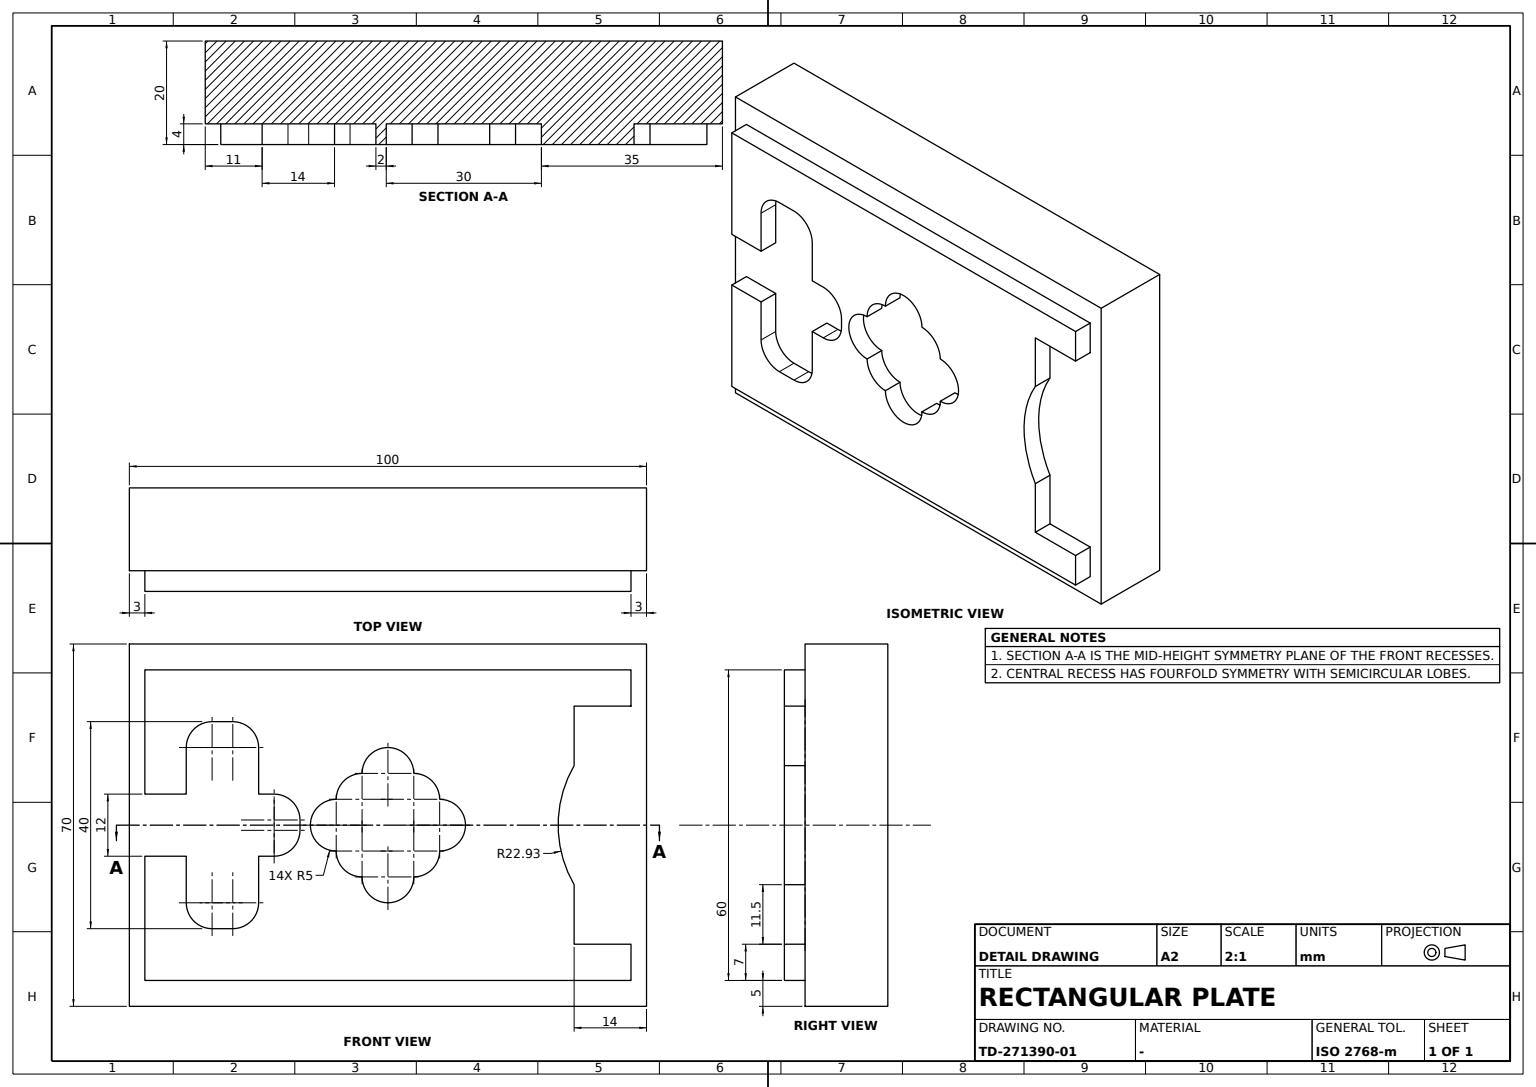
ISO-10303-21;
HEADER;
FILE_DESCRIPTION((''),'2;1');
FILE_NAME('','',(''),(''),'','','');
FILE_SCHEMA(('AUTOMOTIVE_DESIGN'));
ENDSEC;
DATA;
#1=APPLICATION_CONTEXT('');
#2=PRODUCT_CONTEXT('',#1,'mechanical');
#3=PRODUCT('','','',(#2));
#4=PRODUCT_DEFINITION_FORMATION('','',#3);
#5=PRODUCT_DEFINITION_CONTEXT('',#1,'design');
#6=PRODUCT_DEFINITION('','',#4,#5);
#7=PRODUCT_DEFINITION_SHAPE('','',#6);
#8=(LENGTH_UNIT()NAMED_UNIT(*)SI_UNIT(.MILLI.,.METRE.));
#9=(NAMED_UNIT(*)PLANE_ANGLE_UNIT()SI_UNIT($,.RADIAN.));
#10=(NAMED_UNIT(*)SI_UNIT($,.STERADIAN.)SOLID_ANGLE_UNIT());
#11=UNCERTAINTY_MEASURE_WITH_UNIT(LENGTH_MEASURE(0.005),#8,'distance_accuracy_value','');
#12=(GEOMETRIC_REPRESENTATION_CONTEXT(3)GLOBAL_UNCERTAINTY_ASSIGNED_CONTEXT((#11))GLOBAL_UNIT_ASSIGNED_CONTEXT((#8,#9,#10))REPRESENTATION_CONTEXT('',''));
#13=CARTESIAN_POINT('',(-30.,-20.,-20.));
#14=VERTEX_POINT('',#13);
#15=CARTESIAN_POINT('',(-30.,-16.,-20.));
#16=VERTEX_POINT('',#15);
#17=DIRECTION('',(0.,1.,0.));
#18=VECTOR('',#17,1000.);
#19=LINE('',#15,#18);
#20=EDGE_CURVE('',#14,#16,#19,.T.);
#21=ORIENTED_EDGE('',*,*,#20,.F.);
#22=CARTESIAN_POINT('',(-25.,-20.,-15.));
#23=VERTEX_POINT('',#22);
#24=CARTESIAN_POINT('',(-30.,-20.,-15.));
#25=DIRECTION('',(0.,-1.,0.));
#26=DIRECTION('',(1.,0.,0.));
#27=AXIS2_PLACEMENT_3D('',#24,#25,#26);
#28=CIRCLE('',#27,5.);
#29=EDGE_CURVE('',#14,#23,#28,.T.);
#30=ORIENTED_EDGE('',*,*,#29,.T.);
#31=CARTESIAN_POINT('',(-25.,-16.,-15.));
#32=VERTEX_POINT('',#31);
#33=LINE('',#31,#18);
#34=EDGE_CURVE('',#23,#32,#33,.T.);
#35=ORIENTED_EDGE('',*,*,#34,.T.);
#36=CARTESIAN_POINT('',(-30.,-16.,-15.));
#37=AXIS2_PLACEMENT_3D('',#36,#25,#26);
#38=CIRCLE('',#37,5.);
#39=EDGE_CURVE('',#16,#32,#38,.T.);
#40=ORIENTED_EDGE('',*,*,#39,.F.);
#41=EDGE_LOOP('',(#21,#30,#35,#40));
#42=FACE_BOUND('',#41,.T.);
#43=DIRECTION('',(0.,0.,-1.));
#44=AXIS2_PLACEMENT_3D('',#36,#25,#43);
#45=CYLINDRICAL_SURFACE('',#44,5.);
#46=ADVANCED_FACE('',(#42),#45,.F.);
#47=CARTESIAN_POINT('',(-10.,-20.,5.));
#48=VERTEX_POINT('',#47);
#49=CARTESIAN_POINT('',(-10.,-16.,5.));
#50=VERTEX_POINT('',#49);
#51=LINE('',#49,#18);
#52=EDGE_CURVE('',#48,#50,#51,.T.);
#53=ORIENTED_EDGE('',*,*,#52,.T.);
#54=CARTESIAN_POINT('',(-5.,-16.,10.));
#55=VERTEX_POINT('',#54);
#56=CARTESIAN_POINT('',(-5.,-16.,5.));
#57=AXIS2_PLACEMENT_3D('',#56,#17,#26);
#58=CIRCLE('',#57,5.);
#59=EDGE_CURVE('',#50,#55,#58,.T.);
#60=ORIENTED_EDGE('',*,*,#59,.T.);
#61=CARTESIAN_POINT('',(-5.,-20.,10.));
#62=VERTEX_POINT('',#61);
#63=LINE('',#54,#18);
#64=EDGE_CURVE('',#62,#55,#63,.T.);
#65=ORIENTED_EDGE('',*,*,#64,.F.);
#66=CARTESIAN_POINT('',(-5.,-20.,5.));
#67=AXIS2_PLACEMENT_3D('',#66,#25,#26);
#68=CIRCLE('',#67,5.);
#69=EDGE_CURVE('',#62,#48,#68,.T.);
#70=ORIENTED_EDGE('',*,*,#69,.T.);
#71=EDGE_LOOP('',(#53,#60,#65,#70));
#72=FACE_BOUND('',#71,.T.);
#73=AXIS2_PLACEMENT_3D('',#56,#25,#43);
#74=CYLINDRICAL_SURFACE('',#73,5.);
#75=ADVANCED_FACE('',(#72),#74,.F.);
#76=CARTESIAN_POINT('',(36.,-16.,23.));
#77=VERTEX_POINT('',#76);
#78=CARTESIAN_POINT('',(36.,-16.,11.5));
#79=VERTEX_POINT('',#78);
#80=VECTOR('',#43,1000.);
#81=LINE('',#76,#80);
#82=EDGE_CURVE('',#77,#79,#81,.T.);
#83=ORIENTED_EDGE('',*,*,#82,.T.);
#84=CARTESIAN_POINT('',(36.,-16.,-11.5));
#85=VERTEX_POINT('',#84);
#86=CARTESIAN_POINT('',(55.837208,-16.,0.));
#87=AXIS2_PLACEMENT_3D('',#86,#25,#26);
#88=CIRCLE('',#87,22.929562);
#89=EDGE_CURVE('',#79,#85,#88,.T.);
#90=ORIENTED_EDGE('',*,*,#89,.T.);
#91=CARTESIAN_POINT('',(36.,-16.,-23.));
#92=VERTEX_POINT('',#91);
#93=LINE('',#84,#80);
#94=EDGE_CURVE('',#85,#92,#93,.T.);
#95=ORIENTED_EDGE('',*,*,#94,.T.);
#96=CARTESIAN_POINT('',(47.,-16.,-23.));
#97=VERTEX_POINT('',#96);
#98=VECTOR('',#26,1000.);
#99=LINE('',#91,#98);
#100=EDGE_CURVE('',#92,#97,#99,.T.);
#101=ORIENTED_EDGE('',*,*,#100,.T.);
#102=CARTESIAN_POINT('',(47.,-16.,-30.));
#103=VERTEX_POINT('',#102);
#104=DIRECTION('',(0.,0.,1.));
#105=VECTOR('',#104,1000.);
#106=LINE('',#102,#105);
#107=EDGE_CURVE('',#103,#97,#106,.T.);
#108=ORIENTED_EDGE('',*,*,#107,.F.);
#109=CARTESIAN_POINT('',(-47.,-16.,-30.));
#110=VERTEX_POINT('',#109);
#111=LINE('',#109,#98);
#112=EDGE_CURVE('',#110,#103,#111,.T.);
#113=ORIENTED_EDGE('',*,*,#112,.F.);
#114=CARTESIAN_POINT('',(-47.,-16.,-6.));
#115=VERTEX_POINT('',#114);
#116=CARTESIAN_POINT('',(-47.,-16.,30.));
#117=LINE('',#116,#80);
#118=EDGE_CURVE('',#115,#110,#117,.T.);
#119=ORIENTED_EDGE('',*,*,#118,.F.);
#120=CARTESIAN_POINT('',(-39.,-16.,-6.));
#121=VERTEX_POINT('',#120);
#122=LINE('',#114,#98);
#123=EDGE_CURVE('',#115,#121,#122,.T.);
#124=ORIENTED_EDGE('',*,*,#123,.T.);
#125=CARTESIAN_POINT('',(-39.,-16.,-15.));
#126=VERTEX_POINT('',#125);
#127=LINE('',#120,#80);
#128=EDGE_CURVE('',#121,#126,#127,.T.);
#129=ORIENTED_EDGE('',*,*,#128,.T.);
#130=CARTESIAN_POINT('',(-34.,-16.,-20.));
#131=VERTEX_POINT('',#130);
#132=CARTESIAN_POINT('',(-34.,-16.,-15.));
#133=AXIS2_PLACEMENT_3D('',#132,#25,#26);
#134=CIRCLE('',#133,5.);
#135=EDGE_CURVE('',#126,#131,#134,.T.);
#136=ORIENTED_EDGE('',*,*,#135,.T.);
#137=LINE('',#130,#98);
#138=EDGE_CURVE('',#131,#16,#137,.T.);
#139=ORIENTED_EDGE('',*,*,#138,.T.);
#140=ORIENTED_EDGE('',*,*,#39,.T.);
#141=CARTESIAN_POINT('',(-25.,-16.,-6.));
#142=VERTEX_POINT('',#141);
#143=LINE('',#31,#105);
#144=EDGE_CURVE('',#32,#142,#143,.T.);
#145=ORIENTED_EDGE('',*,*,#144,.T.);
#146=CARTESIAN_POINT('',(-22.,-16.,-6.));
#147=VERTEX_POINT('',#146);
#148=LINE('',#141,#98);
#149=EDGE_CURVE('',#142,#147,#148,.T.);
#150=ORIENTED_EDGE('',*,*,#149,.T.);
#151=CARTESIAN_POINT('',(-17.,-16.,-1.));
#152=VERTEX_POINT('',#151);
#153=CARTESIAN_POINT('',(-22.,-16.,-1.));
#154=AXIS2_PLACEMENT_3D('',#153,#25,#26);
#155=CIRCLE('',#154,5.);
#156=EDGE_CURVE('',#147,#152,#155,.T.);
#157=ORIENTED_EDGE('',*,*,#156,.T.);
#158=CARTESIAN_POINT('',(-17.,-16.,1.));
#159=VERTEX_POINT('',#158);
#160=LINE('',#151,#105);
#161=EDGE_CURVE('',#152,#159,#160,.T.);
#162=ORIENTED_EDGE('',*,*,#161,.T.);
#163=CARTESIAN_POINT('',(-22.,-16.,6.));
#164=VERTEX_POINT('',#163);
#165=CARTESIAN_POINT('',(-22.,-16.,1.));
#166=AXIS2_PLACEMENT_3D('',#165,#25,#26);
#167=CIRCLE('',#166,5.);
#168=EDGE_CURVE('',#159,#164,#167,.T.);
#169=ORIENTED_EDGE('',*,*,#168,.T.);
#170=CARTESIAN_POINT('',(-25.,-16.,6.));
#171=VERTEX_POINT('',#170);
#172=DIRECTION('',(-1.,0.,0.));
#173=VECTOR('',#172,1000.);
#174=LINE('',#163,#173);
#175=EDGE_CURVE('',#164,#171,#174,.T.);
#176=ORIENTED_EDGE('',*,*,#175,.T.);
#177=CARTESIAN_POINT('',(-25.,-16.,15.));
#178=VERTEX_POINT('',#177);
#179=LINE('',#170,#105);
#180=EDGE_CURVE('',#171,#178,#179,.T.);
#181=ORIENTED_EDGE('',*,*,#180,.T.);
#182=CARTESIAN_POINT('',(-30.,-16.,20.));
#183=VERTEX_POINT('',#182);
#184=CARTESIAN_POINT('',(-30.,-16.,15.));
#185=AXIS2_PLACEMENT_3D('',#184,#25,#26);
#186=CIRCLE('',#185,5.);
#187=EDGE_CURVE('',#178,#183,#186,.T.);
#188=ORIENTED_EDGE('',*,*,#187,.T.);
#189=CARTESIAN_POINT('',(-34.,-16.,20.));
#190=VERTEX_POINT('',#189);
#191=LINE('',#182,#173);
#192=EDGE_CURVE('',#183,#190,#191,.T.);
#193=ORIENTED_EDGE('',*,*,#192,.T.);
#194=CARTESIAN_POINT('',(-39.,-16.,15.));
#195=VERTEX_POINT('',#194);
#196=CARTESIAN_POINT('',(-34.,-16.,15.));
#197=AXIS2_PLACEMENT_3D('',#196,#25,#26);
#198=CIRCLE('',#197,5.);
#199=EDGE_CURVE('',#190,#195,#198,.T.);
#200=ORIENTED_EDGE('',*,*,#199,.T.);
#201=CARTESIAN_POINT('',(-39.,-16.,6.));
#202=VERTEX_POINT('',#201);
#203=LINE('',#194,#80);
#204=EDGE_CURVE('',#195,#202,#203,.T.);
#205=ORIENTED_EDGE('',*,*,#204,.T.);
#206=CARTESIAN_POINT('',(-47.,-16.,6.));
#207=VERTEX_POINT('',#206);
#208=LINE('',#201,#173);
#209=EDGE_CURVE('',#202,#207,#208,.T.);
#210=ORIENTED_EDGE('',*,*,#209,.T.);
#211=VERTEX_POINT('',#116);
#212=EDGE_CURVE('',#211,#207,#117,.T.);
#213=ORIENTED_EDGE('',*,*,#212,.F.);
#214=CARTESIAN_POINT('',(47.,-16.,30.));
#215=VERTEX_POINT('',#214);
#216=LINE('',#214,#173);
#217=EDGE_CURVE('',#215,#211,#216,.T.);
#218=ORIENTED_EDGE('',*,*,#217,.F.);
#219=CARTESIAN_POINT('',(47.,-16.,23.));
#220=VERTEX_POINT('',#219);
#221=EDGE_CURVE('',#220,#215,#106,.T.);
#222=ORIENTED_EDGE('',*,*,#221,.F.);
#223=LINE('',#219,#173);
#224=EDGE_CURVE('',#220,#77,#223,.T.);
#225=ORIENTED_EDGE('',*,*,#224,.T.);
#226=EDGE_LOOP('',(#83,#90,#95,#101,#108,#113,#119,#124,#129,#136,#139,#140,#145,#150,#157,#162,#169,#176,#181,#188,#193,#200,#205,#210,#213,#218,#222,#225));
#227=FACE_BOUND('',#226,.T.);
#228=CARTESIAN_POINT('',(50.,-16.,35.));
#229=VERTEX_POINT('',#228);
#230=CARTESIAN_POINT('',(-50.,-16.,35.));
#231=VERTEX_POINT('',#230);
#232=LINE('',#228,#173);
#233=EDGE_CURVE('',#229,#231,#232,.T.);
#234=ORIENTED_EDGE('',*,*,#233,.T.);
#235=CARTESIAN_POINT('',(-50.,-16.,-35.));
#236=VERTEX_POINT('',#235);
#237=LINE('',#230,#80);
#238=EDGE_CURVE('',#231,#236,#237,.T.);
#239=ORIENTED_EDGE('',*,*,#238,.T.);
#240=CARTESIAN_POINT('',(50.,-16.,-35.));
#241=VERTEX_POINT('',#240);
#242=LINE('',#235,#98);
#243=EDGE_CURVE('',#236,#241,#242,.T.);
#244=ORIENTED_EDGE('',*,*,#243,.T.);
#245=LINE('',#240,#105);
#246=EDGE_CURVE('',#241,#229,#245,.T.);
#247=ORIENTED_EDGE('',*,*,#246,.T.);
#248=EDGE_LOOP('',(#234,#239,#244,#247));
#249=FACE_BOUND('',#248,.T.);
#250=CARTESIAN_POINT('',(0.,-16.,0.));
#251=AXIS2_PLACEMENT_3D('',#250,#25,#43);
#252=PLANE('',#251);
#253=ADVANCED_FACE('',(#227,#249),#252,.T.);
#254=CARTESIAN_POINT('',(-47.,-20.,-6.));
#255=VERTEX_POINT('',#254);
#256=VECTOR('',#25,1000.);
#257=LINE('',#114,#256);
#258=EDGE_CURVE('',#115,#255,#257,.T.);
#259=ORIENTED_EDGE('',*,*,#258,.F.);
#260=ORIENTED_EDGE('',*,*,#118,.T.);
#261=CARTESIAN_POINT('',(-47.,-20.,-30.));
#262=VERTEX_POINT('',#261);
#263=LINE('',#261,#18);
#264=EDGE_CURVE('',#262,#110,#263,.T.);
#265=ORIENTED_EDGE('',*,*,#264,.F.);
#266=CARTESIAN_POINT('',(-47.,-20.,30.));
#267=LINE('',#266,#80);
#268=EDGE_CURVE('',#255,#262,#267,.T.);
#269=ORIENTED_EDGE('',*,*,#268,.F.);
#270=EDGE_LOOP('',(#259,#260,#265,#269));
#271=FACE_BOUND('',#270,.T.);
#272=AXIS2_PLACEMENT_3D('',#266,#26,#43);
#273=PLANE('',#272);
#274=ADVANCED_FACE('',(#271),#273,.F.);
#275=CARTESIAN_POINT('',(-22.,-20.,-6.));
#276=VERTEX_POINT('',#275);
#277=LINE('',#146,#18);
#278=EDGE_CURVE('',#276,#147,#277,.T.);
#279=ORIENTED_EDGE('',*,*,#278,.F.);
#280=CARTESIAN_POINT('',(-17.,-20.,-1.));
#281=VERTEX_POINT('',#280);
#282=CARTESIAN_POINT('',(-22.,-20.,-1.));
#283=AXIS2_PLACEMENT_3D('',#282,#25,#26);
#284=CIRCLE('',#283,5.);
#285=EDGE_CURVE('',#276,#281,#284,.T.);
#286=ORIENTED_EDGE('',*,*,#285,.T.);
#287=LINE('',#151,#18);
#288=EDGE_CURVE('',#281,#152,#287,.T.);
#289=ORIENTED_EDGE('',*,*,#288,.T.);
#290=ORIENTED_EDGE('',*,*,#156,.F.);
#291=EDGE_LOOP('',(#279,#286,#289,#290));
#292=FACE_BOUND('',#291,.T.);
#293=AXIS2_PLACEMENT_3D('',#153,#25,#43);
#294=CYLINDRICAL_SURFACE('',#293,5.);
#295=ADVANCED_FACE('',(#292),#294,.F.);
#296=CARTESIAN_POINT('',(0.,-20.,-15.));
#297=VERTEX_POINT('',#296);
#298=CARTESIAN_POINT('',(5.,-20.,-10.));
#299=VERTEX_POINT('',#298);
#300=CARTESIAN_POINT('',(0.,-20.,-10.));
#301=AXIS2_PLACEMENT_3D('',#300,#25,#172);
#302=CIRCLE('',#301,5.);
#303=EDGE_CURVE('',#297,#299,#302,.T.);
#304=ORIENTED_EDGE('',*,*,#303,.T.);
#305=CARTESIAN_POINT('',(5.,-16.,-10.));
#306=VERTEX_POINT('',#305);
#307=LINE('',#305,#18);
#308=EDGE_CURVE('',#299,#306,#307,.T.);
#309=ORIENTED_EDGE('',*,*,#308,.T.);
#310=CARTESIAN_POINT('',(0.,-16.,-15.));
#311=VERTEX_POINT('',#310);
#312=CARTESIAN_POINT('',(0.,-16.,-10.));
#313=AXIS2_PLACEMENT_3D('',#312,#17,#172);
#314=CIRCLE('',#313,5.);
#315=EDGE_CURVE('',#306,#311,#314,.T.);
#316=ORIENTED_EDGE('',*,*,#315,.T.);
#317=LINE('',#310,#256);
#318=EDGE_CURVE('',#311,#297,#317,.T.);
#319=ORIENTED_EDGE('',*,*,#318,.T.);
#320=EDGE_LOOP('',(#304,#309,#316,#319));
#321=FACE_BOUND('',#320,.T.);
#322=AXIS2_PLACEMENT_3D('',#312,#25,#43);
#323=CYLINDRICAL_SURFACE('',#322,5.);
#324=ADVANCED_FACE('',(#321),#323,.F.);
#325=CARTESIAN_POINT('',(-50.,0.,35.));
#326=VERTEX_POINT('',#325);
#327=CARTESIAN_POINT('',(-50.,0.,-35.));
#328=VERTEX_POINT('',#327);
#329=LINE('',#325,#80);
#330=EDGE_CURVE('',#326,#328,#329,.T.);
#331=ORIENTED_EDGE('',*,*,#330,.T.);
#332=LINE('',#235,#18);
#333=EDGE_CURVE('',#236,#328,#332,.T.);
#334=ORIENTED_EDGE('',*,*,#333,.F.);
#335=ORIENTED_EDGE('',*,*,#238,.F.);
#336=LINE('',#230,#18);
#337=EDGE_CURVE('',#231,#326,#336,.T.);
#338=ORIENTED_EDGE('',*,*,#337,.T.);
#339=EDGE_LOOP('',(#331,#334,#335,#338));
#340=FACE_BOUND('',#339,.T.);
#341=AXIS2_PLACEMENT_3D('',#230,#26,#43);
#342=PLANE('',#341);
#343=ADVANCED_FACE('',(#340),#342,.F.);
#344=CARTESIAN_POINT('',(50.,0.,-35.));
#345=VERTEX_POINT('',#344);
#346=CARTESIAN_POINT('',(50.,0.,35.));
#347=VERTEX_POINT('',#346);
#348=LINE('',#344,#105);
#349=EDGE_CURVE('',#345,#347,#348,.T.);
#350=ORIENTED_EDGE('',*,*,#349,.T.);
#351=LINE('',#228,#18);
#352=EDGE_CURVE('',#229,#347,#351,.T.);
#353=ORIENTED_EDGE('',*,*,#352,.F.);
#354=ORIENTED_EDGE('',*,*,#246,.F.);
#355=LINE('',#240,#18);
#356=EDGE_CURVE('',#241,#345,#355,.T.);
#357=ORIENTED_EDGE('',*,*,#356,.T.);
#358=EDGE_LOOP('',(#350,#353,#354,#357));
#359=FACE_BOUND('',#358,.T.);
#360=AXIS2_PLACEMENT_3D('',#240,#172,#104);
#361=PLANE('',#360);
#362=ADVANCED_FACE('',(#359),#361,.F.);
#363=CARTESIAN_POINT('',(36.,-20.,23.));
#364=VERTEX_POINT('',#363);
#365=LINE('',#76,#18);
#366=EDGE_CURVE('',#364,#77,#365,.T.);
#367=ORIENTED_EDGE('',*,*,#366,.T.);
#368=ORIENTED_EDGE('',*,*,#224,.F.);
#369=CARTESIAN_POINT('',(47.,-20.,23.));
#370=VERTEX_POINT('',#369);
#371=LINE('',#219,#256);
#372=EDGE_CURVE('',#220,#370,#371,.T.);
#373=ORIENTED_EDGE('',*,*,#372,.T.);
#374=LINE('',#369,#173);
#375=EDGE_CURVE('',#370,#364,#374,.T.);
#376=ORIENTED_EDGE('',*,*,#375,.T.);
#377=EDGE_LOOP('',(#367,#368,#373,#376));
#378=FACE_BOUND('',#377,.T.);
#379=AXIS2_PLACEMENT_3D('',#219,#104,#26);
#380=PLANE('',#379);
#381=ADVANCED_FACE('',(#378),#380,.F.);
#382=CARTESIAN_POINT('',(36.,-20.,-11.5));
#383=VERTEX_POINT('',#382);
#384=LINE('',#84,#18);
#385=EDGE_CURVE('',#383,#85,#384,.T.);
#386=ORIENTED_EDGE('',*,*,#385,.T.);
#387=ORIENTED_EDGE('',*,*,#89,.F.);
#388=CARTESIAN_POINT('',(36.,-20.,11.5));
#389=VERTEX_POINT('',#388);
#390=LINE('',#78,#18);
#391=EDGE_CURVE('',#389,#79,#390,.T.);
#392=ORIENTED_EDGE('',*,*,#391,.F.);
#393=CARTESIAN_POINT('',(55.837208,-20.,0.));
#394=AXIS2_PLACEMENT_3D('',#393,#25,#26);
#395=CIRCLE('',#394,22.929562);
#396=EDGE_CURVE('',#389,#383,#395,.T.);
#397=ORIENTED_EDGE('',*,*,#396,.T.);
#398=EDGE_LOOP('',(#386,#387,#392,#397));
#399=FACE_BOUND('',#398,.T.);
#400=AXIS2_PLACEMENT_3D('',#86,#25,#43);
#401=CYLINDRICAL_SURFACE('',#400,22.929562);
#402=ADVANCED_FACE('',(#399),#401,.F.);
#403=ORIENTED_EDGE('',*,*,#315,.F.);
#404=CARTESIAN_POINT('',(10.,-16.,-5.));
#405=VERTEX_POINT('',#404);
#406=CARTESIAN_POINT('',(5.,-16.,-5.));
#407=AXIS2_PLACEMENT_3D('',#406,#17,#172);
#408=CIRCLE('',#407,5.);
#409=EDGE_CURVE('',#405,#306,#408,.T.);
#410=ORIENTED_EDGE('',*,*,#409,.F.);
#411=CARTESIAN_POINT('',(10.,-16.,5.));
#412=VERTEX_POINT('',#411);
#413=CARTESIAN_POINT('',(10.,-16.,0.));
#414=AXIS2_PLACEMENT_3D('',#413,#17,#43);
#415=CIRCLE('',#414,5.);
#416=EDGE_CURVE('',#412,#405,#415,.T.);
#417=ORIENTED_EDGE('',*,*,#416,.F.);
#418=CARTESIAN_POINT('',(5.,-16.,10.));
#419=VERTEX_POINT('',#418);
#420=CARTESIAN_POINT('',(5.,-16.,5.));
#421=AXIS2_PLACEMENT_3D('',#420,#17,#172);
#422=CIRCLE('',#421,5.);
#423=EDGE_CURVE('',#419,#412,#422,.T.);
#424=ORIENTED_EDGE('',*,*,#423,.F.);
#425=CARTESIAN_POINT('',(0.,-16.,10.));
#426=AXIS2_PLACEMENT_3D('',#425,#17,#26);
#427=CIRCLE('',#426,5.);
#428=EDGE_CURVE('',#55,#419,#427,.T.);
#429=ORIENTED_EDGE('',*,*,#428,.F.);
#430=ORIENTED_EDGE('',*,*,#59,.F.);
#431=CARTESIAN_POINT('',(-10.,-16.,-5.));
#432=VERTEX_POINT('',#431);
#433=CARTESIAN_POINT('',(-10.,-16.,0.));
#434=AXIS2_PLACEMENT_3D('',#433,#17,#104);
#435=CIRCLE('',#434,5.);
#436=EDGE_CURVE('',#432,#50,#435,.T.);
#437=ORIENTED_EDGE('',*,*,#436,.F.);
#438=CARTESIAN_POINT('',(-5.,-16.,-10.));
#439=VERTEX_POINT('',#438);
#440=CARTESIAN_POINT('',(-5.,-16.,-5.));
#441=AXIS2_PLACEMENT_3D('',#440,#17,#26);
#442=CIRCLE('',#441,5.);
#443=EDGE_CURVE('',#439,#432,#442,.T.);
#444=ORIENTED_EDGE('',*,*,#443,.F.);
#445=EDGE_CURVE('',#311,#439,#314,.T.);
#446=ORIENTED_EDGE('',*,*,#445,.F.);
#447=EDGE_LOOP('',(#403,#410,#417,#424,#429,#430,#437,#444,#446));
#448=FACE_BOUND('',#447,.T.);
#449=CARTESIAN_POINT('',(-7.5,-16.,-2.5));
#450=AXIS2_PLACEMENT_3D('',#449,#25,#43);
#451=PLANE('',#450);
#452=ADVANCED_FACE('',(#448),#451,.T.);
#453=CARTESIAN_POINT('',(-17.,-20.,1.));
#454=VERTEX_POINT('',#453);
#455=LINE('',#158,#18);
#456=EDGE_CURVE('',#454,#159,#455,.T.);
#457=ORIENTED_EDGE('',*,*,#456,.T.);
#458=ORIENTED_EDGE('',*,*,#161,.F.);
#459=ORIENTED_EDGE('',*,*,#288,.F.);
#460=LINE('',#280,#105);
#461=EDGE_CURVE('',#281,#454,#460,.T.);
#462=ORIENTED_EDGE('',*,*,#461,.T.);
#463=EDGE_LOOP('',(#457,#458,#459,#462));
#464=FACE_BOUND('',#463,.T.);
#465=AXIS2_PLACEMENT_3D('',#151,#26,#43);
#466=PLANE('',#465);
#467=ADVANCED_FACE('',(#464),#466,.F.);
#468=CARTESIAN_POINT('',(-39.,-20.,-15.));
#469=VERTEX_POINT('',#468);
#470=LINE('',#125,#18);
#471=EDGE_CURVE('',#469,#126,#470,.T.);
#472=ORIENTED_EDGE('',*,*,#471,.T.);
#473=ORIENTED_EDGE('',*,*,#128,.F.);
#474=CARTESIAN_POINT('',(-39.,-20.,-6.));
#475=VERTEX_POINT('',#474);
#476=LINE('',#120,#18);
#477=EDGE_CURVE('',#475,#121,#476,.T.);
#478=ORIENTED_EDGE('',*,*,#477,.F.);
#479=LINE('',#474,#80);
#480=EDGE_CURVE('',#475,#469,#479,.T.);
#481=ORIENTED_EDGE('',*,*,#480,.T.);
#482=EDGE_LOOP('',(#472,#473,#478,#481));
#483=FACE_BOUND('',#482,.T.);
#484=AXIS2_PLACEMENT_3D('',#120,#172,#104);
#485=PLANE('',#484);
#486=ADVANCED_FACE('',(#483),#485,.F.);
#487=CARTESIAN_POINT('',(10.,-20.,-5.));
#488=VERTEX_POINT('',#487);
#489=CARTESIAN_POINT('',(10.,-20.,5.));
#490=VERTEX_POINT('',#489);
#491=CARTESIAN_POINT('',(10.,-20.,0.));
#492=AXIS2_PLACEMENT_3D('',#491,#25,#43);
#493=CIRCLE('',#492,5.);
#494=EDGE_CURVE('',#488,#490,#493,.T.);
#495=ORIENTED_EDGE('',*,*,#494,.T.);
#496=LINE('',#411,#18);
#497=EDGE_CURVE('',#490,#412,#496,.T.);
#498=ORIENTED_EDGE('',*,*,#497,.T.);
#499=ORIENTED_EDGE('',*,*,#416,.T.);
#500=LINE('',#404,#18);
#501=EDGE_CURVE('',#488,#405,#500,.T.);
#502=ORIENTED_EDGE('',*,*,#501,.F.);
#503=EDGE_LOOP('',(#495,#498,#499,#502));
#504=FACE_BOUND('',#503,.T.);
#505=AXIS2_PLACEMENT_3D('',#413,#25,#43);
#506=CYLINDRICAL_SURFACE('',#505,5.);
#507=ADVANCED_FACE('',(#504),#506,.F.);
#508=ORIENTED_EDGE('',*,*,#112,.T.);
#509=CARTESIAN_POINT('',(47.,-20.,-30.));
#510=VERTEX_POINT('',#509);
#511=LINE('',#509,#18);
#512=EDGE_CURVE('',#510,#103,#511,.T.);
#513=ORIENTED_EDGE('',*,*,#512,.F.);
#514=LINE('',#261,#98);
#515=EDGE_CURVE('',#262,#510,#514,.T.);
#516=ORIENTED_EDGE('',*,*,#515,.F.);
#517=ORIENTED_EDGE('',*,*,#264,.T.);
#518=EDGE_LOOP('',(#508,#513,#516,#517));
#519=FACE_BOUND('',#518,.T.);
#520=AXIS2_PLACEMENT_3D('',#261,#104,#26);
#521=PLANE('',#520);
#522=ADVANCED_FACE('',(#519),#521,.F.);
#523=ORIENTED_EDGE('',*,*,#258,.T.);
#524=LINE('',#254,#98);
#525=EDGE_CURVE('',#255,#475,#524,.T.);
#526=ORIENTED_EDGE('',*,*,#525,.T.);
#527=ORIENTED_EDGE('',*,*,#477,.T.);
#528=ORIENTED_EDGE('',*,*,#123,.F.);
#529=EDGE_LOOP('',(#523,#526,#527,#528));
#530=FACE_BOUND('',#529,.T.);
#531=AXIS2_PLACEMENT_3D('',#114,#43,#172);
#532=PLANE('',#531);
#533=ADVANCED_FACE('',(#530),#532,.F.);
#534=ORIENTED_EDGE('',*,*,#337,.F.);
#535=ORIENTED_EDGE('',*,*,#233,.F.);
#536=ORIENTED_EDGE('',*,*,#352,.T.);
#537=LINE('',#346,#173);
#538=EDGE_CURVE('',#347,#326,#537,.T.);
#539=ORIENTED_EDGE('',*,*,#538,.T.);
#540=EDGE_LOOP('',(#534,#535,#536,#539));
#541=FACE_BOUND('',#540,.T.);
#542=AXIS2_PLACEMENT_3D('',#228,#43,#172);
#543=PLANE('',#542);
#544=ADVANCED_FACE('',(#541),#543,.F.);
#545=CARTESIAN_POINT('',(5.,-20.,10.));
#546=VERTEX_POINT('',#545);
#547=CARTESIAN_POINT('',(5.,-20.,5.));
#548=AXIS2_PLACEMENT_3D('',#547,#25,#172);
#549=CIRCLE('',#548,5.);
#550=EDGE_CURVE('',#490,#546,#549,.T.);
#551=ORIENTED_EDGE('',*,*,#550,.T.);
#552=LINE('',#418,#18);
#553=EDGE_CURVE('',#546,#419,#552,.T.);
#554=ORIENTED_EDGE('',*,*,#553,.T.);
#555=ORIENTED_EDGE('',*,*,#423,.T.);
#556=ORIENTED_EDGE('',*,*,#497,.F.);
#557=EDGE_LOOP('',(#551,#554,#555,#556));
#558=FACE_BOUND('',#557,.T.);
#559=AXIS2_PLACEMENT_3D('',#420,#25,#43);
#560=CYLINDRICAL_SURFACE('',#559,5.);
#561=ADVANCED_FACE('',(#558),#560,.F.);
#562=CARTESIAN_POINT('',(-39.,-20.,6.));
#563=VERTEX_POINT('',#562);
#564=LINE('',#201,#18);
#565=EDGE_CURVE('',#563,#202,#564,.T.);
#566=ORIENTED_EDGE('',*,*,#565,.F.);
#567=CARTESIAN_POINT('',(-47.,-20.,6.));
#568=VERTEX_POINT('',#567);
#569=LINE('',#562,#173);
#570=EDGE_CURVE('',#563,#568,#569,.T.);
#571=ORIENTED_EDGE('',*,*,#570,.T.);
#572=LINE('',#206,#256);
#573=EDGE_CURVE('',#207,#568,#572,.T.);
#574=ORIENTED_EDGE('',*,*,#573,.F.);
#575=ORIENTED_EDGE('',*,*,#209,.F.);
#576=EDGE_LOOP('',(#566,#571,#574,#575));
#577=FACE_BOUND('',#576,.T.);
#578=AXIS2_PLACEMENT_3D('',#201,#104,#26);
#579=PLANE('',#578);
#580=ADVANCED_FACE('',(#577),#579,.F.);
#581=ORIENTED_EDGE('',*,*,#515,.T.);
#582=CARTESIAN_POINT('',(47.,-20.,-23.));
#583=VERTEX_POINT('',#582);
#584=LINE('',#509,#105);
#585=EDGE_CURVE('',#510,#583,#584,.T.);
#586=ORIENTED_EDGE('',*,*,#585,.T.);
#587=CARTESIAN_POINT('',(36.,-20.,-23.));
#588=VERTEX_POINT('',#587);
#589=LINE('',#587,#98);
#590=EDGE_CURVE('',#588,#583,#589,.T.);
#591=ORIENTED_EDGE('',*,*,#590,.F.);
#592=LINE('',#382,#80);
#593=EDGE_CURVE('',#383,#588,#592,.T.);
#594=ORIENTED_EDGE('',*,*,#593,.F.);
#595=ORIENTED_EDGE('',*,*,#396,.F.);
#596=LINE('',#363,#80);
#597=EDGE_CURVE('',#364,#389,#596,.T.);
#598=ORIENTED_EDGE('',*,*,#597,.F.);
#599=ORIENTED_EDGE('',*,*,#375,.F.);
#600=CARTESIAN_POINT('',(47.,-20.,30.));
#601=VERTEX_POINT('',#600);
#602=EDGE_CURVE('',#370,#601,#584,.T.);
#603=ORIENTED_EDGE('',*,*,#602,.T.);
#604=VERTEX_POINT('',#266);
#605=LINE('',#600,#173);
#606=EDGE_CURVE('',#601,#604,#605,.T.);
#607=ORIENTED_EDGE('',*,*,#606,.T.);
#608=EDGE_CURVE('',#604,#568,#267,.T.);
#609=ORIENTED_EDGE('',*,*,#608,.T.);
#610=ORIENTED_EDGE('',*,*,#570,.F.);
#611=CARTESIAN_POINT('',(-39.,-20.,15.));
#612=VERTEX_POINT('',#611);
#613=LINE('',#611,#80);
#614=EDGE_CURVE('',#612,#563,#613,.T.);
#615=ORIENTED_EDGE('',*,*,#614,.F.);
#616=CARTESIAN_POINT('',(-34.,-20.,20.));
#617=VERTEX_POINT('',#616);
#618=CARTESIAN_POINT('',(-34.,-20.,15.));
#619=AXIS2_PLACEMENT_3D('',#618,#25,#26);
#620=CIRCLE('',#619,5.);
#621=EDGE_CURVE('',#617,#612,#620,.T.);
#622=ORIENTED_EDGE('',*,*,#621,.F.);
#623=CARTESIAN_POINT('',(-30.,-20.,20.));
#624=VERTEX_POINT('',#623);
#625=LINE('',#623,#173);
#626=EDGE_CURVE('',#624,#617,#625,.T.);
#627=ORIENTED_EDGE('',*,*,#626,.F.);
#628=CARTESIAN_POINT('',(-25.,-20.,15.));
#629=VERTEX_POINT('',#628);
#630=CARTESIAN_POINT('',(-30.,-20.,15.));
#631=AXIS2_PLACEMENT_3D('',#630,#25,#26);
#632=CIRCLE('',#631,5.);
#633=EDGE_CURVE('',#629,#624,#632,.T.);
#634=ORIENTED_EDGE('',*,*,#633,.F.);
#635=CARTESIAN_POINT('',(-25.,-20.,6.));
#636=VERTEX_POINT('',#635);
#637=LINE('',#635,#105);
#638=EDGE_CURVE('',#636,#629,#637,.T.);
#639=ORIENTED_EDGE('',*,*,#638,.F.);
#640=CARTESIAN_POINT('',(-22.,-20.,6.));
#641=VERTEX_POINT('',#640);
#642=LINE('',#640,#173);
#643=EDGE_CURVE('',#641,#636,#642,.T.);
#644=ORIENTED_EDGE('',*,*,#643,.F.);
#645=CARTESIAN_POINT('',(-22.,-20.,1.));
#646=AXIS2_PLACEMENT_3D('',#645,#25,#26);
#647=CIRCLE('',#646,5.);
#648=EDGE_CURVE('',#454,#641,#647,.T.);
#649=ORIENTED_EDGE('',*,*,#648,.F.);
#650=ORIENTED_EDGE('',*,*,#461,.F.);
#651=ORIENTED_EDGE('',*,*,#285,.F.);
#652=CARTESIAN_POINT('',(-25.,-20.,-6.));
#653=VERTEX_POINT('',#652);
#654=LINE('',#652,#98);
#655=EDGE_CURVE('',#653,#276,#654,.T.);
#656=ORIENTED_EDGE('',*,*,#655,.F.);
#657=LINE('',#22,#105);
#658=EDGE_CURVE('',#23,#653,#657,.T.);
#659=ORIENTED_EDGE('',*,*,#658,.F.);
#660=ORIENTED_EDGE('',*,*,#29,.F.);
#661=CARTESIAN_POINT('',(-34.,-20.,-20.));
#662=VERTEX_POINT('',#661);
#663=LINE('',#661,#98);
#664=EDGE_CURVE('',#662,#14,#663,.T.);
#665=ORIENTED_EDGE('',*,*,#664,.F.);
#666=CARTESIAN_POINT('',(-34.,-20.,-15.));
#667=AXIS2_PLACEMENT_3D('',#666,#25,#26);
#668=CIRCLE('',#667,5.);
#669=EDGE_CURVE('',#469,#662,#668,.T.);
#670=ORIENTED_EDGE('',*,*,#669,.F.);
#671=ORIENTED_EDGE('',*,*,#480,.F.);
#672=ORIENTED_EDGE('',*,*,#525,.F.);
#673=ORIENTED_EDGE('',*,*,#268,.T.);
#674=EDGE_LOOP('',(#581,#586,#591,#594,#595,#598,#599,#603,#607,#609,#610,#615,#622,#627,#634,#639,#644,#649,#650,#651,#656,#659,#660,#665,#670,#671,#672,#673));
#675=FACE_BOUND('',#674,.T.);
#676=CARTESIAN_POINT('',(0.,-20.,10.));
#677=AXIS2_PLACEMENT_3D('',#676,#25,#26);
#678=CIRCLE('',#677,5.);
#679=EDGE_CURVE('',#546,#62,#678,.T.);
#680=ORIENTED_EDGE('',*,*,#679,.F.);
#681=ORIENTED_EDGE('',*,*,#550,.F.);
#682=ORIENTED_EDGE('',*,*,#494,.F.);
#683=CARTESIAN_POINT('',(5.,-20.,-5.));
#684=AXIS2_PLACEMENT_3D('',#683,#25,#172);
#685=CIRCLE('',#684,5.);
#686=EDGE_CURVE('',#299,#488,#685,.T.);
#687=ORIENTED_EDGE('',*,*,#686,.F.);
#688=ORIENTED_EDGE('',*,*,#303,.F.);
#689=CARTESIAN_POINT('',(-5.,-20.,-10.));
#690=VERTEX_POINT('',#689);
#691=EDGE_CURVE('',#690,#297,#302,.T.);
#692=ORIENTED_EDGE('',*,*,#691,.F.);
#693=CARTESIAN_POINT('',(-10.,-20.,-5.));
#694=VERTEX_POINT('',#693);
#695=CARTESIAN_POINT('',(-5.,-20.,-5.));
#696=AXIS2_PLACEMENT_3D('',#695,#25,#26);
#697=CIRCLE('',#696,5.);
#698=EDGE_CURVE('',#694,#690,#697,.T.);
#699=ORIENTED_EDGE('',*,*,#698,.F.);
#700=CARTESIAN_POINT('',(-10.,-20.,0.));
#701=AXIS2_PLACEMENT_3D('',#700,#25,#104);
#702=CIRCLE('',#701,5.);
#703=EDGE_CURVE('',#48,#694,#702,.T.);
#704=ORIENTED_EDGE('',*,*,#703,.F.);
#705=ORIENTED_EDGE('',*,*,#69,.F.);
#706=EDGE_LOOP('',(#680,#681,#682,#687,#688,#692,#699,#704,#705));
#707=FACE_BOUND('',#706,.T.);
#708=CARTESIAN_POINT('',(0.,-20.,0.));
#709=AXIS2_PLACEMENT_3D('',#708,#25,#43);
#710=PLANE('',#709);
#711=ADVANCED_FACE('',(#675,#707),#710,.T.);
#712=ORIENTED_EDGE('',*,*,#20,.T.);
#713=ORIENTED_EDGE('',*,*,#138,.F.);
#714=LINE('',#130,#18);
#715=EDGE_CURVE('',#662,#131,#714,.T.);
#716=ORIENTED_EDGE('',*,*,#715,.F.);
#717=ORIENTED_EDGE('',*,*,#664,.T.);
#718=EDGE_LOOP('',(#712,#713,#716,#717));
#719=FACE_BOUND('',#718,.T.);
#720=AXIS2_PLACEMENT_3D('',#130,#43,#172);
#721=PLANE('',#720);
#722=ADVANCED_FACE('',(#719),#721,.F.);
#723=ORIENTED_EDGE('',*,*,#633,.T.);
#724=LINE('',#182,#18);
#725=EDGE_CURVE('',#624,#183,#724,.T.);
#726=ORIENTED_EDGE('',*,*,#725,.T.);
#727=ORIENTED_EDGE('',*,*,#187,.F.);
#728=LINE('',#177,#18);
#729=EDGE_CURVE('',#629,#178,#728,.T.);
#730=ORIENTED_EDGE('',*,*,#729,.F.);
#731=EDGE_LOOP('',(#723,#726,#727,#730));
#732=FACE_BOUND('',#731,.T.);
#733=AXIS2_PLACEMENT_3D('',#184,#25,#43);
#734=CYLINDRICAL_SURFACE('',#733,5.);
#735=ADVANCED_FACE('',(#732),#734,.F.);
#736=ORIENTED_EDGE('',*,*,#703,.T.);
#737=LINE('',#431,#18);
#738=EDGE_CURVE('',#694,#432,#737,.T.);
#739=ORIENTED_EDGE('',*,*,#738,.T.);
#740=ORIENTED_EDGE('',*,*,#436,.T.);
#741=ORIENTED_EDGE('',*,*,#52,.F.);
#742=EDGE_LOOP('',(#736,#739,#740,#741));
#743=FACE_BOUND('',#742,.T.);
#744=AXIS2_PLACEMENT_3D('',#433,#25,#43);
#745=CYLINDRICAL_SURFACE('',#744,5.);
#746=ADVANCED_FACE('',(#743),#745,.F.);
#747=ORIENTED_EDGE('',*,*,#349,.F.);
#748=LINE('',#327,#98);
#749=EDGE_CURVE('',#328,#345,#748,.T.);
#750=ORIENTED_EDGE('',*,*,#749,.F.);
#751=ORIENTED_EDGE('',*,*,#330,.F.);
#752=ORIENTED_EDGE('',*,*,#538,.F.);
#753=EDGE_LOOP('',(#747,#750,#751,#752));
#754=FACE_BOUND('',#753,.T.);
#755=CARTESIAN_POINT('',(0.,0.,0.));
#756=AXIS2_PLACEMENT_3D('',#755,#25,#43);
#757=PLANE('',#756);
#758=ADVANCED_FACE('',(#754),#757,.F.);
#759=ORIENTED_EDGE('',*,*,#725,.F.);
#760=ORIENTED_EDGE('',*,*,#626,.T.);
#761=LINE('',#189,#18);
#762=EDGE_CURVE('',#617,#190,#761,.T.);
#763=ORIENTED_EDGE('',*,*,#762,.T.);
#764=ORIENTED_EDGE('',*,*,#192,.F.);
#765=EDGE_LOOP('',(#759,#760,#763,#764));
#766=FACE_BOUND('',#765,.T.);
#767=AXIS2_PLACEMENT_3D('',#182,#104,#26);
#768=PLANE('',#767);
#769=ADVANCED_FACE('',(#766),#768,.F.);
#770=LINE('',#438,#18);
#771=EDGE_CURVE('',#690,#439,#770,.T.);
#772=ORIENTED_EDGE('',*,*,#771,.T.);
#773=ORIENTED_EDGE('',*,*,#443,.T.);
#774=ORIENTED_EDGE('',*,*,#738,.F.);
#775=ORIENTED_EDGE('',*,*,#698,.T.);
#776=EDGE_LOOP('',(#772,#773,#774,#775));
#777=FACE_BOUND('',#776,.T.);
#778=AXIS2_PLACEMENT_3D('',#440,#25,#43);
#779=CYLINDRICAL_SURFACE('',#778,5.);
#780=ADVANCED_FACE('',(#777),#779,.F.);
#781=ORIENTED_EDGE('',*,*,#565,.T.);
#782=ORIENTED_EDGE('',*,*,#204,.F.);
#783=LINE('',#194,#18);
#784=EDGE_CURVE('',#612,#195,#783,.T.);
#785=ORIENTED_EDGE('',*,*,#784,.F.);
#786=ORIENTED_EDGE('',*,*,#614,.T.);
#787=EDGE_LOOP('',(#781,#782,#785,#786));
#788=FACE_BOUND('',#787,.T.);
#789=AXIS2_PLACEMENT_3D('',#194,#172,#104);
#790=PLANE('',#789);
#791=ADVANCED_FACE('',(#788),#790,.F.);
#792=ORIENTED_EDGE('',*,*,#356,.F.);
#793=ORIENTED_EDGE('',*,*,#243,.F.);
#794=ORIENTED_EDGE('',*,*,#333,.T.);
#795=ORIENTED_EDGE('',*,*,#749,.T.);
#796=EDGE_LOOP('',(#792,#793,#794,#795));
#797=FACE_BOUND('',#796,.T.);
#798=AXIS2_PLACEMENT_3D('',#235,#104,#26);
#799=PLANE('',#798);
#800=ADVANCED_FACE('',(#797),#799,.F.);
#801=ORIENTED_EDGE('',*,*,#573,.T.);
#802=ORIENTED_EDGE('',*,*,#608,.F.);
#803=LINE('',#266,#18);
#804=EDGE_CURVE('',#604,#211,#803,.T.);
#805=ORIENTED_EDGE('',*,*,#804,.T.);
#806=ORIENTED_EDGE('',*,*,#212,.T.);
#807=EDGE_LOOP('',(#801,#802,#805,#806));
#808=FACE_BOUND('',#807,.T.);
#809=ADVANCED_FACE('',(#808),#273,.F.);
#810=ORIENTED_EDGE('',*,*,#691,.T.);
#811=ORIENTED_EDGE('',*,*,#318,.F.);
#812=ORIENTED_EDGE('',*,*,#445,.T.);
#813=ORIENTED_EDGE('',*,*,#771,.F.);
#814=EDGE_LOOP('',(#810,#811,#812,#813));
#815=FACE_BOUND('',#814,.T.);
#816=ADVANCED_FACE('',(#815),#323,.F.);
#817=ORIENTED_EDGE('',*,*,#593,.T.);
#818=LINE('',#91,#18);
#819=EDGE_CURVE('',#588,#92,#818,.T.);
#820=ORIENTED_EDGE('',*,*,#819,.T.);
#821=ORIENTED_EDGE('',*,*,#94,.F.);
#822=ORIENTED_EDGE('',*,*,#385,.F.);
#823=EDGE_LOOP('',(#817,#820,#821,#822));
#824=FACE_BOUND('',#823,.T.);
#825=AXIS2_PLACEMENT_3D('',#84,#172,#104);
#826=PLANE('',#825);
#827=ADVANCED_FACE('',(#824),#826,.F.);
#828=ORIENTED_EDGE('',*,*,#175,.F.);
#829=LINE('',#163,#18);
#830=EDGE_CURVE('',#641,#164,#829,.T.);
#831=ORIENTED_EDGE('',*,*,#830,.F.);
#832=ORIENTED_EDGE('',*,*,#643,.T.);
#833=LINE('',#170,#18);
#834=EDGE_CURVE('',#636,#171,#833,.T.);
#835=ORIENTED_EDGE('',*,*,#834,.T.);
#836=EDGE_LOOP('',(#828,#831,#832,#835));
#837=FACE_BOUND('',#836,.T.);
#838=AXIS2_PLACEMENT_3D('',#163,#104,#26);
#839=PLANE('',#838);
#840=ADVANCED_FACE('',(#837),#839,.F.);
#841=ORIENTED_EDGE('',*,*,#784,.T.);
#842=ORIENTED_EDGE('',*,*,#199,.F.);
#843=ORIENTED_EDGE('',*,*,#762,.F.);
#844=ORIENTED_EDGE('',*,*,#621,.T.);
#845=EDGE_LOOP('',(#841,#842,#843,#844));
#846=FACE_BOUND('',#845,.T.);
#847=AXIS2_PLACEMENT_3D('',#196,#25,#43);
#848=CYLINDRICAL_SURFACE('',#847,5.);
#849=ADVANCED_FACE('',(#846),#848,.F.);
#850=ORIENTED_EDGE('',*,*,#648,.T.);
#851=ORIENTED_EDGE('',*,*,#830,.T.);
#852=ORIENTED_EDGE('',*,*,#168,.F.);
#853=ORIENTED_EDGE('',*,*,#456,.F.);
#854=EDGE_LOOP('',(#850,#851,#852,#853));
#855=FACE_BOUND('',#854,.T.);
#856=AXIS2_PLACEMENT_3D('',#165,#25,#43);
#857=CYLINDRICAL_SURFACE('',#856,5.);
#858=ADVANCED_FACE('',(#855),#857,.F.);
#859=ORIENTED_EDGE('',*,*,#669,.T.);
#860=ORIENTED_EDGE('',*,*,#715,.T.);
#861=ORIENTED_EDGE('',*,*,#135,.F.);
#862=ORIENTED_EDGE('',*,*,#471,.F.);
#863=EDGE_LOOP('',(#859,#860,#861,#862));
#864=FACE_BOUND('',#863,.T.);
#865=AXIS2_PLACEMENT_3D('',#132,#25,#43);
#866=CYLINDRICAL_SURFACE('',#865,5.);
#867=ADVANCED_FACE('',(#864),#866,.F.);
#868=ORIENTED_EDGE('',*,*,#428,.T.);
#869=ORIENTED_EDGE('',*,*,#553,.F.);
#870=ORIENTED_EDGE('',*,*,#679,.T.);
#871=ORIENTED_EDGE('',*,*,#64,.T.);
#872=EDGE_LOOP('',(#868,#869,#870,#871));
#873=FACE_BOUND('',#872,.T.);
#874=AXIS2_PLACEMENT_3D('',#425,#25,#43);
#875=CYLINDRICAL_SURFACE('',#874,5.);
#876=ADVANCED_FACE('',(#873),#875,.F.);
#877=ORIENTED_EDGE('',*,*,#391,.T.);
#878=ORIENTED_EDGE('',*,*,#82,.F.);
#879=ORIENTED_EDGE('',*,*,#366,.F.);
#880=ORIENTED_EDGE('',*,*,#597,.T.);
#881=EDGE_LOOP('',(#877,#878,#879,#880));
#882=FACE_BOUND('',#881,.T.);
#883=AXIS2_PLACEMENT_3D('',#76,#172,#104);
#884=PLANE('',#883);
#885=ADVANCED_FACE('',(#882),#884,.F.);
#886=ORIENTED_EDGE('',*,*,#308,.F.);
#887=ORIENTED_EDGE('',*,*,#686,.T.);
#888=ORIENTED_EDGE('',*,*,#501,.T.);
#889=ORIENTED_EDGE('',*,*,#409,.T.);
#890=EDGE_LOOP('',(#886,#887,#888,#889));
#891=FACE_BOUND('',#890,.T.);
#892=AXIS2_PLACEMENT_3D('',#406,#25,#43);
#893=CYLINDRICAL_SURFACE('',#892,5.);
#894=ADVANCED_FACE('',(#891),#893,.F.);
#895=LINE('',#600,#18);
#896=EDGE_CURVE('',#601,#215,#895,.T.);
#897=ORIENTED_EDGE('',*,*,#896,.F.);
#898=ORIENTED_EDGE('',*,*,#602,.F.);
#899=ORIENTED_EDGE('',*,*,#372,.F.);
#900=ORIENTED_EDGE('',*,*,#221,.T.);
#901=EDGE_LOOP('',(#897,#898,#899,#900));
#902=FACE_BOUND('',#901,.T.);
#903=AXIS2_PLACEMENT_3D('',#509,#172,#104);
#904=PLANE('',#903);
#905=ADVANCED_FACE('',(#902),#904,.F.);
#906=ORIENTED_EDGE('',*,*,#804,.F.);
#907=ORIENTED_EDGE('',*,*,#606,.F.);
#908=ORIENTED_EDGE('',*,*,#896,.T.);
#909=ORIENTED_EDGE('',*,*,#217,.T.);
#910=EDGE_LOOP('',(#906,#907,#908,#909));
#911=FACE_BOUND('',#910,.T.);
#912=AXIS2_PLACEMENT_3D('',#600,#43,#172);
#913=PLANE('',#912);
#914=ADVANCED_FACE('',(#911),#913,.F.);
#915=LINE('',#96,#256);
#916=EDGE_CURVE('',#97,#583,#915,.T.);
#917=ORIENTED_EDGE('',*,*,#916,.T.);
#918=ORIENTED_EDGE('',*,*,#585,.F.);
#919=ORIENTED_EDGE('',*,*,#512,.T.);
#920=ORIENTED_EDGE('',*,*,#107,.T.);
#921=EDGE_LOOP('',(#917,#918,#919,#920));
#922=FACE_BOUND('',#921,.T.);
#923=ADVANCED_FACE('',(#922),#904,.F.);
#924=ORIENTED_EDGE('',*,*,#144,.F.);
#925=ORIENTED_EDGE('',*,*,#34,.F.);
#926=ORIENTED_EDGE('',*,*,#658,.T.);
#927=LINE('',#141,#18);
#928=EDGE_CURVE('',#653,#142,#927,.T.);
#929=ORIENTED_EDGE('',*,*,#928,.T.);
#930=EDGE_LOOP('',(#924,#925,#926,#929));
#931=FACE_BOUND('',#930,.T.);
#932=AXIS2_PLACEMENT_3D('',#31,#26,#43);
#933=PLANE('',#932);
#934=ADVANCED_FACE('',(#931),#933,.F.);
#935=ORIENTED_EDGE('',*,*,#655,.T.);
#936=ORIENTED_EDGE('',*,*,#278,.T.);
#937=ORIENTED_EDGE('',*,*,#149,.F.);
#938=ORIENTED_EDGE('',*,*,#928,.F.);
#939=EDGE_LOOP('',(#935,#936,#937,#938));
#940=FACE_BOUND('',#939,.T.);
#941=AXIS2_PLACEMENT_3D('',#141,#43,#172);
#942=PLANE('',#941);
#943=ADVANCED_FACE('',(#940),#942,.F.);
#944=ORIENTED_EDGE('',*,*,#590,.T.);
#945=ORIENTED_EDGE('',*,*,#916,.F.);
#946=ORIENTED_EDGE('',*,*,#100,.F.);
#947=ORIENTED_EDGE('',*,*,#819,.F.);
#948=EDGE_LOOP('',(#944,#945,#946,#947));
#949=FACE_BOUND('',#948,.T.);
#950=AXIS2_PLACEMENT_3D('',#91,#43,#172);
#951=PLANE('',#950);
#952=ADVANCED_FACE('',(#949),#951,.F.);
#953=ORIENTED_EDGE('',*,*,#180,.F.);
#954=ORIENTED_EDGE('',*,*,#834,.F.);
#955=ORIENTED_EDGE('',*,*,#638,.T.);
#956=ORIENTED_EDGE('',*,*,#729,.T.);
#957=EDGE_LOOP('',(#953,#954,#955,#956));
#958=FACE_BOUND('',#957,.T.);
#959=AXIS2_PLACEMENT_3D('',#170,#26,#43);
#960=PLANE('',#959);
#961=ADVANCED_FACE('',(#958),#960,.F.);
#962=CLOSED_SHELL('',(#46,#75,#253,#274,#295,#324,#343,#362,#381,#402,#452,#467,#486,#507,#522,#533,#544,#561,#580,#711,#722,#735,#746,#758,#769,#780,#791,#800,#809,#816,#827,#840,#849,#858,#867,#876,#885,#894,#905,#914,#923,#934,#943,#952,#961));
#963=MANIFOLD_SOLID_BREP('',#962);
#964=ADVANCED_BREP_SHAPE_REPRESENTATION('',(#963),#12);
#965=SHAPE_DEFINITION_REPRESENTATION(#7,#964);
ENDSEC;
END-ISO-10303-21;
